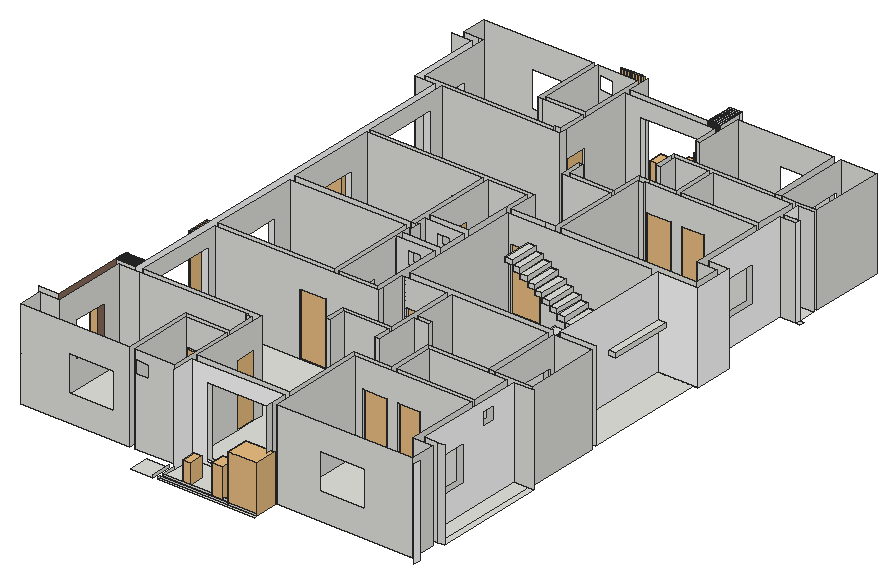
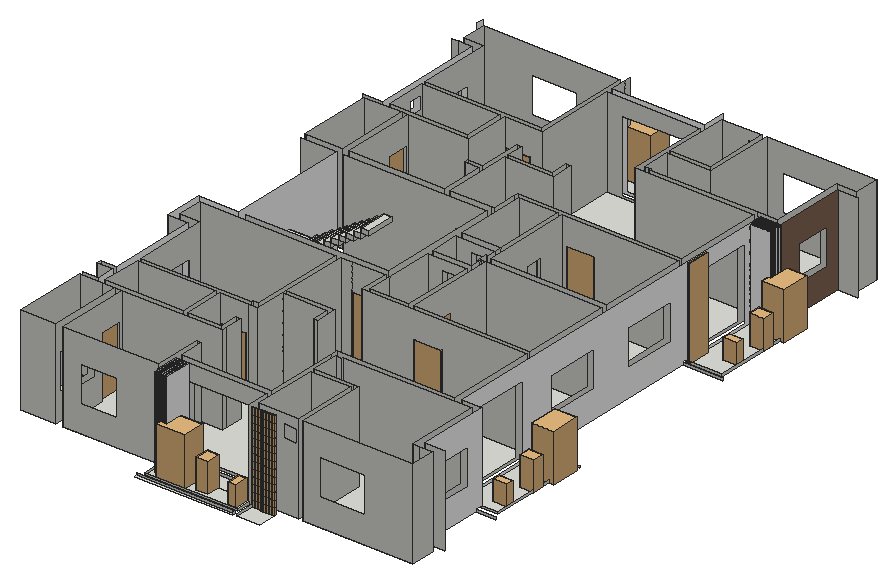
# SketchUp Ruby script. Lengths in inches.
U = 1.inch
M = Sketchup.active_model
def pt(a) = Geom::Point3d.new(a.map { |v| v * U })
def face(e, loops, mat)
  f = e.add_face(loops[0].map { |a| pt(a) })
  loops[1..].each { |l| e.add_face(l.map { |a| pt(a) }).erase! }
  f.material = f.back_material = mat if mat
  f
end
# faces: each face lists its corners as indices into pts; further lists are holes
def faces(e, pts, list, mat = nil) = list.each { |f| face(e, (f[0].is_a?(Array) ? f : [f]).map { |l| l.map { |i| pts[i] } }, mat) }
# xy, xz, yz: faces in a plane at the given z, y or x. An outline is a flat list of corners, or four numbers for a rectangle; further outlines are holes
def ring(l) = l.size == 4 ? [[l[0], l[1]], [l[2], l[1]], [l[2], l[3]], [l[0], l[3]]] : l.each_slice(2).to_a
def flat(e, list, mat, &to3) = list.each { |f| face(e, (f[0].is_a?(Array) ? f : [f]).map { |l| ring(l).map { |u, v| to3.(u, v) } }, mat) }
def xy(e, z, list, mat = nil) = flat(e, list, mat) { |x, y| [x, y, z] }
def xz(e, y, list, mat = nil) = flat(e, list, mat) { |x, z| [x, y, z] }
def yz(e, x, list, mat = nil) = flat(e, list, mat) { |y, z| [x, y, z] }
def lines(e, pts, list) = list.each { |a, b| e.add_line(pt(pts[a]), pt(pts[b])) }
# prism: a flat outline (further loops are holes) pulled along v
def prism(e, loops, v, mat = nil)
  f = face(e, loops, mat); d = Geom::Vector3d.new(v.map { |x| x * U })
  f.pushpull(f.normal.samedirection?(d) ? d.length : -d.length)
end
def box(e, o, s, mat = nil) = prism(e, [[o, [o[0] + s[0], o[1], o[2]], [o[0] + s[0], o[1] + s[1], o[2]], [o[0], o[1] + s[1], o[2]]]], [0, 0, s[2]], mat)
def at(x, y, z, deg = 0) = Geom::Transformation.translation(pt([x, y, z])) * Geom::Transformation.rotation(ORIGIN, Z_AXIS, deg.degrees)
def axes(o, x, y, z) = Geom::Transformation.new([*x, 0, *y, 0, *z, 0, *pt(o).to_a, 1])
def part(name) = M.definitions.add(name)
# library, detail: a bought-in or finely detailed component or shape, given as its bounding box
def library(name, o, s) = part(name).tap { |d| box(d.entities, o, s) }
def detail(e, o, s) = box(e.add_group.entities, o, s)
def put(e, d, t, mat = nil) = e.add_instance(d, t).tap { |i| i.material = mat if mat }
def group(e, t, mat = nil) = e.add_group.tap { |g| g.transformation = t; g.material = mat if mat }.entities
root = M.entities
M.materials.add("Manhattan Creative Coating ML 1016B 24.75cm").color = [255, 255, 255]
M.materials.add("Wintan - wpa36452 29.79cm").color = [255, 255, 255]
M.materials.add("Wood Planks C01 100cm").color = [136, 107, 89]
c1 = library("Door 243 053",[-21.6,-2.79,-0.07],[43.2,5.58,82.64])
c2 = library("Potted Plant 13",[-10,-7.28,0],[18.93,15.17,39.22])
c3 = library("Potted Plant 50-12",[-6.11,-5.26,0],[11.24,10.56,13.41])
c4 = library("Potted Plant 02",[-16.98,-19.78,0],[30.04,38.68,37.52])
c5 = part("Rectangular column")
box(c5.entities,[0,16,0],[27,1,119.8])
box(c5.entities,[0,3.56,0],[27,1,120])
box(c5.entities,[0,1.78,0],[27,1,120])
box(c5.entities,[0,14.22,0],[27,1,119.8])
box(c5.entities,[0,5.33,0],[27,1,120])
box(c5.entities,[0,7.11,0],[27,1,120])
box(c5.entities,[0,10.67,0],[27,1,120.2])
box(c5.entities,[0,12.44,0],[27,1,119.8])
box(c5.entities,[0,0,0],[27,1,120])
xy(c5.entities,0,[[0,8.89,27,9.89]])
xy(c5.entities,120,[[0,8.89,27,9.89]])
xz(c5.entities,8.89,[[0,0,27,120]])
xz(c5.entities,9.89,[[0,0,27,120]])
yz(c5.entities,0,[[8.89,0,9.89,120]],"Wintan - wpa36452 29.79cm")
yz(c5.entities,27,[[8.89,0,9.89,120]])
c6 = part("Stair tread \#1")
box(c6.entities,[0,0,0],[10,39,7])
c7 = part("Stair tread")
box(c7.entities,[0,0,0],[10,39,7])
c8 = part("Group\#9")
box(c8.entities,[100,0,63],[49,84,7])
box(c8.entities,[0,45,0],[20,39,7])
put(c8.entities,c6,at(50,45,28))
put(c8.entities,c6,at(20,45,7))
put(c8.entities,c6,at(90,45,56))
put(c8.entities,c6,at(70,45,42))
put(c8.entities,c6,at(40,45,21))
put(c8.entities,c6,at(60,45,35))
put(c8.entities,c6,at(30,45,14))
put(c8.entities,c6,at(80,45,49))
put(c8.entities,c7,at(90,0,70))
put(c8.entities,c7,at(10,0,126))
put(c8.entities,c7,at(60,0,91))
put(c8.entities,c7,at(30,0,112))
put(c8.entities,c7,at(50,0,98))
put(c8.entities,c7,at(70,0,84))
put(c8.entities,c7,at(80,0,77))
put(c8.entities,c7,at(40,0,105))
put(c8.entities,c7,at(0,0,133))
put(c8.entities,c7,at(20,0,119))
c9 = part("Decorative grille insert")
p = [[0.961,0,5],[0.961,0,4.995]]
lines(c9.entities,p,[[0,1]])
detail(c9.entities,[0,0,0],[4.12,1.8,10])
c10 = part("Group\#25")
put(c10.entities,c9,at(0,0,0))
put(c10.entities,c9,at(4.12,0,0))
put(c10.entities,c9,at(8.24,0,0))
put(c10.entities,c9,at(12.36,0,0))
put(c10.entities,c9,at(16.48,0,0))
put(c10.entities,c9,at(20.61,0,0))
put(c10.entities,c9,at(24.73,0,0))
put(c10.entities,c9,at(28.85,0,0))
put(c10.entities,c9,at(0,0,10))
put(c10.entities,c9,at(28.85,0,10))
put(c10.entities,c9,at(24.73,0,10))
put(c10.entities,c9,at(20.61,0,10))
put(c10.entities,c9,at(12.36,0,10))
put(c10.entities,c9,at(16.48,0,10))
put(c10.entities,c9,at(4.12,0,10))
put(c10.entities,c9,at(8.24,0,10))
put(c10.entities,c9,at(0,0,20))
put(c10.entities,c9,at(28.85,0,20))
put(c10.entities,c9,at(24.73,0,20))
put(c10.entities,c9,at(20.61,0,20))
put(c10.entities,c9,at(12.36,0,20))
put(c10.entities,c9,at(16.48,0,20))
put(c10.entities,c9,at(4.12,0,20))
put(c10.entities,c9,at(8.24,0,20))
put(c10.entities,c9,at(0,0,30))
put(c10.entities,c9,at(28.85,0,30))
put(c10.entities,c9,at(24.73,0,30))
put(c10.entities,c9,at(20.61,0,30))
put(c10.entities,c9,at(12.36,0,30))
put(c10.entities,c9,at(16.48,0,30))
put(c10.entities,c9,at(4.12,0,30))
put(c10.entities,c9,at(8.24,0,30))
put(c10.entities,c9,at(0,0,40))
put(c10.entities,c9,at(28.85,0,40))
put(c10.entities,c9,at(24.73,0,40))
put(c10.entities,c9,at(20.61,0,40))
put(c10.entities,c9,at(12.36,0,40))
put(c10.entities,c9,at(16.48,0,40))
put(c10.entities,c9,at(4.12,0,40))
put(c10.entities,c9,at(8.24,0,40))
put(c10.entities,c9,at(0,0,50))
put(c10.entities,c9,at(28.85,0,50))
put(c10.entities,c9,at(24.73,0,50))
put(c10.entities,c9,at(20.61,0,50))
put(c10.entities,c9,at(12.36,0,50))
put(c10.entities,c9,at(16.48,0,50))
put(c10.entities,c9,at(4.12,0,50))
put(c10.entities,c9,at(8.24,0,50))
put(c10.entities,c9,at(0,0,60))
put(c10.entities,c9,at(28.85,0,60))
put(c10.entities,c9,at(24.73,0,60))
put(c10.entities,c9,at(20.61,0,60))
put(c10.entities,c9,at(12.36,0,60))
put(c10.entities,c9,at(16.48,0,60))
put(c10.entities,c9,at(4.12,0,60))
put(c10.entities,c9,at(8.24,0,60))
put(c10.entities,c9,at(0,0,70))
put(c10.entities,c9,at(28.85,0,70))
put(c10.entities,c9,at(24.73,0,70))
put(c10.entities,c9,at(20.61,0,70))
put(c10.entities,c9,at(12.36,0,70))
put(c10.entities,c9,at(16.48,0,70))
put(c10.entities,c9,at(4.12,0,70))
put(c10.entities,c9,at(8.24,0,70))
put(c10.entities,c9,at(0,0,80))
put(c10.entities,c9,at(28.85,0,80))
put(c10.entities,c9,at(24.73,0,80))
put(c10.entities,c9,at(20.61,0,80))
put(c10.entities,c9,at(12.36,0,80))
put(c10.entities,c9,at(16.48,0,80))
put(c10.entities,c9,at(4.12,0,80))
put(c10.entities,c9,at(8.24,0,80))
put(c10.entities,c9,at(0,0,90))
put(c10.entities,c9,at(28.85,0,90))
put(c10.entities,c9,at(24.73,0,90))
put(c10.entities,c9,at(20.61,0,90))
put(c10.entities,c9,at(12.36,0,90))
put(c10.entities,c9,at(16.48,0,90))
put(c10.entities,c9,at(4.12,0,90))
put(c10.entities,c9,at(8.24,0,90))
put(c10.entities,c9,at(0,0,100))
put(c10.entities,c9,at(28.85,0,100))
put(c10.entities,c9,at(24.73,0,100))
put(c10.entities,c9,at(20.61,0,100))
put(c10.entities,c9,at(12.36,0,100))
put(c10.entities,c9,at(16.48,0,100))
put(c10.entities,c9,at(4.12,0,100))
put(c10.entities,c9,at(8.24,0,100))
put(c10.entities,c9,at(0,0,110))
put(c10.entities,c9,at(28.85,0,110))
put(c10.entities,c9,at(24.73,0,110))
put(c10.entities,c9,at(20.61,0,110))
put(c10.entities,c9,at(12.36,0,110))
put(c10.entities,c9,at(16.48,0,110))
put(c10.entities,c9,at(4.12,0,110))
put(c10.entities,c9,at(8.24,0,110))
put(c10.entities,c9,at(0,0,120))
put(c10.entities,c9,at(28.85,0,120))
put(c10.entities,c9,at(24.73,0,120))
put(c10.entities,c9,at(20.61,0,120))
put(c10.entities,c9,at(12.36,0,120))
put(c10.entities,c9,at(16.48,0,120))
put(c10.entities,c9,at(4.12,0,120))
put(c10.entities,c9,at(8.24,0,120))
c11 = library("Group1606\#2",[0.89,0.19,0],[2.1,4.18,2.5])
xy(root,126,[[1975.05,473.67,2005.02,500.67],[2011.02,473.67,2141.52,476.67],[2011.02,482.67,2135.52,530.62],[1798.02,509.67,1945.02,509.67,1945.02,602.67,1954.02,602.67,1954.02,596.67,1951.02,596.67,1951.02,509.67,2005.02,509.67,2005.02,596.67,1978.02,596.67,1978.02,602.67,2005.02,602.67,2005.02,605.67,2011.02,605.67,2011.02,635.67,2005.02,635.67,2005.02,638.67,1997.02,638.67,1997.02,641.67,1825.02,641.67,1825.02,542.67,1798.02,542.67],[2141.52,509.67,2324.52,509.67,2324.52,542.67,2297.52,542.67,2297.52,641.67,2228.52,641.67,2228.52,647.67,2198.52,647.67,2198.52,641.67,2184.02,641.67,2184.02,647.67,2152.02,647.67,2152.02,641.67,2141.52,641.67],
  [2011.02,539.67,2135.52,539.67,2135.52,647.67,2186.52,647.67,2186.52,707.67,2267.52,707.67,2267.52,710.67,2276.52,710.67,2276.52,740.67,2267.52,740.67,2267.52,806.67,2138.52,806.67,2138.52,749.67,2158.52,749.67,2158.52,743.67,2138.52,743.67,2138.52,686.67,2132.52,686.67,2132.52,709.17,2072.52,709.17,2072.52,686.67,2066.52,686.67,2066.52,715.17,2132.52,715.17,2132.52,806.67,2117.52,806.67,2117.52,815.67,2078.52,815.67,2078.52,806.67,2072.52,806.67,2072.52,767.67,1852.02,767.67,1852.02,647.67,2011.02,647.67],[2306.52,551.67,2324.52,701.67],[2324.52,551.67,2333.52,701.67],[1795.02,643.17,1816.02,643.17,1816.02,647.67,1843.02,647.67,1843.02,772.17,1795.02,772.17],[2192.52,647.67,2297.52,701.67],
  [2066.52,686.67,2072.52,686.67,2072.52,709.17,2132.52,709.17,2132.52,686.67,2138.52,686.67,2138.52,743.67,2158.52,743.67,2158.52,749.67,2138.52,749.67,2138.52,806.67,2132.52,806.67,2132.52,715.17,2066.52,715.17],[2276.52,707.67,2324.52,806.67],[2324.52,707.67,2327.52,806.67],[1966.02,767.67,2002.02,767.67,2002.02,773.67,2008.02,773.67,2008.02,809.67,2014.02,809.67,2014.02,833.67,2008.02,833.67,2008.02,893.67,1852.02,893.67,1852.02,773.67,1966.02,773.67],[2014.02,773.67,2066.52,869.67],
  [2066.52,806.67,2075.52,806.67,2075.52,980.67,2078.52,980.67,2078.52,989.67,2072.52,989.67,2072.52,1028.67,2002.02,1028.67,2002.02,1022.67,2008.02,1022.67,2008.02,986.67,2014.02,986.67,2014.02,1022.67,2066.52,1022.67,2066.52,926.67,2014.02,926.67,2014.02,962.67,2008.02,962.67,2008.02,902.67,2014.02,902.67,2014.02,917.67,2066.52,917.67,2066.52,878.67,2014.02,878.67,2014.02,869.67,2066.52,869.67],[2075.52,815.67,2207.52,815.67,2207.52,887.67,2267.52,887.67,2267.52,896.67,2138.52,896.67,2138.52,980.67,2117.52,980.67,2117.52,989.67,2078.52,989.67,2078.52,980.67,2075.52,980.67],[2276.52,815.67,2324.52,980.67],[2014.02,878.67,2066.52,878.67,2066.52,917.67,2014.02,917.67,2014.02,905.17,2017.02,905.17,2017.02,891.17,2014.02,891.17],[2143.41,896.68,2143.67,896.68,2143.92,896.76,2144.15,896.89,2144.33,897.08,2144.45,897.31,2144.52,897.56,2144.51,897.82,2144.44,898.07,2144.31,898.3,2144.12,898.48,2143.89,898.6,2143.64,898.67,2143.38,898.66,2143.125,898.59,2142.9,898.46,2142.72,898.27,2142.59,898.04,2142.53,897.79,2142.53,897.53,2142.61,897.28,2142.74,897.05,2142.93,896.87,2143.16,896.74],
  [1852.02,902.67,2008.02,902.67,2008.02,962.67,2014.02,962.67,2014.02,986.67,2008.02,986.67,2008.02,1022.67,2002.02,1022.67,2002.02,1028.67,1966.02,1028.67,1966.02,1022.67,1852.02,1022.67],[2014.02,926.67,2066.52,1022.67],[2143.41,933.68,2143.67,933.68,2143.92,933.76,2144.15,933.89,2144.33,934.08,2144.45,934.31,2144.52,934.56,2144.51,934.82,2144.44,935.07,2144.31,935.3,2144.12,935.48,2143.89,935.6,2143.64,935.67,2143.38,935.66,2143.125,935.59,2142.9,935.46,2142.72,935.27,2142.59,935.04,2142.53,934.79,2142.53,934.53,2142.61,934.28,2142.74,934.05,2142.93,933.87,2143.16,933.74],[2132.52,980.67,2330.52,980.67,2330.52,1022.67,2321.52,1022.67,2321.52,989.67,2138.52,989.67,2138.52,1118.67,2132.52,1118.67],[2072.52,989.67,2132.52,989.67,2132.52,1081.17,2066.52,1081.17,2066.52,1109.67,2072.52,1109.67,2072.52,1087.17,2132.52,1087.17,2132.52,1127.67,2149.02,1127.67,2149.02,1121.67,2146.52,1121.67,2146.52,1118.67,2138.52,1118.67,2138.52,989.67,2321.52,989.67,2321.52,1022.67,2294.52,1022.67,2294.52,1121.67,2225.52,1121.67,2225.52,1127.67,2195.52,1127.67,2195.52,1121.67,2181.02,1121.67,2181.02,1127.67,2183.52,1127.67,2183.52,1181.67,2138.52,1181.67,2138.52,1157.67,2132.52,1157.67,2132.52,1187.67,2267.52,1187.67,2267.52,1190.67,2276.52,1190.67,2276.52,1220.67,2267.52,1220.67,2267.52,1286.67,2138.52,1286.67,2138.52,1223.67,2132.52,1223.67,2132.52,1256.67,2011.02,1256.67,2011.02,1148.67,1852.02,1148.67,1852.02,1028.67,2072.52,1028.67],
  [1852.02,1022.67,1966.02,1028.67],[2294.52,1022.67,2330.52,1022.67,2330.52,1031.67,2303.52,1031.67,2303.52,1151.7,2324.52,1151.7,2324.52,1157.7,2303.52,1157.7,2303.52,1181.67,2294.52,1181.67],[1795.02,1024.17,1843.02,1148.67],[2189.52,1127.67,2294.52,1181.67],[2324.52,1151.7,2330.52,1157.7],
  [1825.02,1154.67,1997.02,1154.67,1997.02,1157.67,2005.02,1157.67,2005.02,1160.17,2011.02,1160.17,2011.02,1190.17,2005.02,1190.17,2005.02,1193.67,1978.02,1193.67,1978.02,1199.67,1954.02,1199.67,1954.02,1193.67,1945.02,1193.67,1945.02,1286.67,1798.02,1286.67,1798.02,1253.67,1825.02,1253.67],[2303.52,1157.7,2324.52,1181.67],[2276.52,1187.67,2324.52,1286.67],[1951.02,1199.67,2005.02,1286.67],[2011.02,1265.67,2132.52,1286.67],
  [2011.02,1286.67,2132.52,1286.67,2132.52,1295.67,2135.52,1295.67,2135.52,1313.67,2011.02,1313.67],[1975.05,1295.67,2005.02,1322.67],[2011.02,1319.67,2141.52,1322.67]])
xz(root,476.67,[[2011.02,126,2141.52,129]])
xz(root,482.67,[[2011.02,126,2135.52,129]])
xz(root,509.67,[[[1798.02,126,1945.02,246],[1863.02,162,1923.02,210]],[[1951.02,126,2005.02,246],[1953.02,216,1970.52,234]],[[2141.52,126,2324.52,246],[2199.52,162,2259.52,210]]])
xz(root,530.62,[[[2011.02,126,2135.52,246],[2031.27,129,2115.27,225]]],"Manhattan Creative Coating ML 1016B 24.75cm")
xz(root,539.67,[[[2011.02,126,2135.52,246],[2031.27,129,2115.27,225]]])
xz(root,542.67,[[1798.02,126,1825.02,246],[2297.52,126,2324.52,246]])
xz(root,551.67,[[1789.02,126,1816.02,246],[2306.52,126,2324.52,246],[2324.52,126,2333.52,246]])
xz(root,596.67,[[1951.02,126,1954.02,126,1954.02,210,1978.02,210,1978.02,126,2005.02,126,2005.02,246,1951.02,246]])
xz(root,602.67,[[1945.02,126,1945.02,246,2005.02,246,2005.02,126,1978.02,126,1978.02,210,1954.02,210,1954.02,126]])
xz(root,605.67,[[2005.02,126,2011.02,210]])
xz(root,635.67,[[2005.02,126,2011.02,210]])
xz(root,637.17,[[1789.02,126,1816.02,129]])
xz(root,638.67,[[1997.02,126,2005.02,246]])
xz(root,641.67,[[1825.02,126,1852.02,246],[1852.02,126,1997.02,246],[2141.52,126,2152.02,126,2152.02,210,2184.02,210,2184.02,126,2198.52,126,2198.52,210,2228.52,210,2228.52,126,2297.52,126,2297.52,246,2141.52,246]])
xz(root,643.17,[[1795.02,126,1816.02,129]])
xz(root,647.67,[[1816.02,126,1843.02,246],[1852.02,126,2011.02,246],[2135.52,126,2135.52,246,2186.52,246,2186.52,126,2184.02,126,2184.02,210,2152.02,210,2152.02,126],[2192.52,126,2192.52,246,2297.52,246,2297.52,126,2228.52,126,2228.52,210,2198.52,210,2198.52,126]])
xz(root,686.67,[[2066.52,126,2072.52,246],[2132.52,126,2138.52,246]])
xz(root,701.67,[[2192.52,126,2297.52,246],[2306.52,126,2333.52,246]])
xz(root,707.67,[[2186.52,126,2267.52,246],[2267.52,126,2276.52,246],[2276.52,126,2327.52,246]])
xz(root,709.17,[[2072.52,126,2132.52,246]])
xz(root,710.67,[[2267.52,126,2276.52,210]])
xz(root,715.17,[[2066.52,126,2132.52,246]])
xz(root,740.67,[[2267.52,126,2276.52,210]])
xz(root,743.67,[[2138.52,126,2158.52,246]])
xz(root,749.67,[[2138.52,126,2158.52,246]])
xz(root,767.67,[[1852.02,126,1966.02,126,1966.02,210,2002.02,210,2002.02,126,2072.52,126,2072.52,246,1852.02,246]])
xz(root,772.17,[[1795.02,126,1843.02,129]])
xz(root,773.67,[[1852.02,126,1852.02,246,2008.02,246,2008.02,126,2002.02,126,2002.02,210,1966.02,210,1966.02,126],[2014.02,126,2066.52,246]])
xz(root,778.17,[[1789.02,126,1843.02,129]])
xz(root,806.67,[[2072.52,126,2075.52,246],[2075.52,126,2078.52,126,2078.52,210,2117.52,210,2117.52,126,2132.52,126,2132.52,246,2075.52,246],[2138.52,126,2267.52,246],[2276.52,126,2324.52,246],[2324.52,126,2327.52,246]])
xz(root,809.67,[[2008.02,126,2014.02,210]])
xz(root,815.67,[[2075.52,126,2075.52,246,2267.52,246,2267.52,126,2117.52,126,2117.52,210,2078.52,210,2078.52,126],[2276.52,126,2324.52,246]])
xz(root,833.67,[[2008.02,126,2014.02,210]])
xz(root,869.67,[[[2014.02,126,2066.52,246],[2029.77,216,2047.27,234]]])
xz(root,878.67,[[[2014.02,126,2066.52,246],[2029.77,216,2047.27,234]]])
xz(root,891.17,[[2014.02,126,2017.02,246]])
xz(root,893.67,[[1852.02,126,2008.02,246]])
xz(root,902.67,[[1852.02,126,2008.02,246],[2008.02,126,2014.02,246]])
xz(root,905.17,[[2014.02,126,2017.02,246]])
xz(root,917.67,[[[2014.02,126,2066.52,246],[2029.77,216,2047.27,234]]])
xz(root,926.67,[[[2014.02,126,2066.52,246],[2029.77,216,2047.27,234]]])
xz(root,962.67,[[2008.02,126,2014.02,210]])
xz(root,980.67,[[2075.52,126,2078.52,126,2078.52,210,2117.52,210,2117.52,126,2267.52,126,2267.52,246,2075.52,246]])
xz(root,980.67,[[2276.52,126,2330.52,246]],"Manhattan Creative Coating ML 1016B 24.75cm")
xz(root,986.67,[[2008.02,126,2014.02,210]])
xz(root,989.67,[[2072.52,126,2072.52,246,2117.52,246,2117.52,210,2078.52,210,2078.52,126],[2117.52,126,2132.52,246],[2138.52,126,2321.52,246]])
xz(root,1018.17,[[1789.02,126,1843.02,129]])
xz(root,1022.67,[[1852.02,126,1966.02,126,1966.02,210,2002.02,210,2002.02,126,2008.02,126,2008.02,246,1852.02,246],[2014.02,126,2066.52,246],[2294.52,126,2321.52,246]])
xz(root,1024.17,[[1795.02,126,1843.02,129]])
xz(root,1028.67,[[1852.02,126,1852.02,246,2072.52,246,2072.52,126,2002.02,126,2002.02,210,1966.02,210,1966.02,126]])
xz(root,1031.67,[[2303.52,126,2330.52,246]])
xz(root,1081.17,[[2066.52,126,2132.52,246]])
xz(root,1087.17,[[2072.52,126,2132.52,246]])
xz(root,1109.67,[[2066.52,126,2072.52,246]])
xz(root,1118.67,[[2138.52,126,2146.52,246]])
xz(root,1121.67,[[2146.52,126,2149.02,126,2149.02,210,2181.02,210,2181.02,126,2195.52,126,2195.52,210,2225.52,210,2225.52,126,2294.52,126,2294.52,246,2146.52,246]])
xz(root,1127.67,[[2132.52,126,2146.52,246],[2146.52,126,2146.52,246,2183.52,246,2183.52,126,2181.02,126,2181.02,210,2149.02,210,2149.02,126],[2189.52,126,2189.52,246,2294.52,246,2294.52,126,2225.52,126,2225.52,210,2195.52,210,2195.52,126]])
xz(root,1148.67,[[1795.02,126,1816.02,129],[1816.02,126,1843.02,246],[1852.02,126,2011.02,246]])
xz(root,1151.7,[[2303.52,126,2324.52,246]])
xz(root,1154.67,[[1825.02,126,1997.02,246]])
xz(root,1157.67,[[1997.02,126,2005.02,246],[2132.52,126,2138.52,246]])
xz(root,1157.7,[[2303.52,126,2324.52,246]])
xz(root,1159.17,[[1789.02,126,1816.02,129]])
xz(root,1160.17,[[2005.02,126,2011.02,210]])
xz(root,1181.67,[[2138.52,126,2183.52,246],[2189.52,126,2294.52,246],[2303.52,126,2324.52,246]])
xz(root,1187.67,[[2132.52,126,2267.52,246],[2267.52,126,2276.52,246],[2276.52,126,2294.52,246],[2294.52,126,2324.52,246]])
xz(root,1190.17,[[2005.02,126,2011.02,210]])
xz(root,1190.67,[[2267.52,126,2276.52,210]])
xz(root,1193.67,[[1945.02,126,1951.02,246],[1951.02,126,1954.02,126,1954.02,210,1978.02,210,1978.02,126,2005.02,126,2005.02,246,1951.02,246]])
xz(root,1199.67,[[1951.02,126,1951.02,246,2005.02,246,2005.02,126,1978.02,126,1978.02,210,1954.02,210,1954.02,126]])
xz(root,1220.67,[[2267.52,126,2276.52,210]])
xz(root,1223.67,[[2132.52,126,2138.52,246]])
xz(root,1244.67,[[1789.02,126,1816.02,246]])
xz(root,1253.67,[[1798.02,126,1816.02,246],[1816.02,126,1825.02,246]])
xz(root,1256.67,[[[2011.02,126,2132.52,246],[2031.27,129,2115.27,225]]])
xz(root,1265.67,[[[2011.02,126,2132.52,246],[2031.27,129,2115.27,225]]])
xz(root,1286.67,[[[1798.02,126,1945.02,246],[1863.02,162,1923.02,210]],[[1951.02,126,2005.02,246],[1953.02,216,1970.52,234]],[[2138.52,126,2267.52,246],[2195.52,162,2243.52,210]],[2276.52,126,2324.52,246]])
xz(root,1313.67,[[2011.02,126,2135.52,129]])
xz(root,1319.67,[[2011.02,126,2141.52,129]])
yz(root,1795.02,[[643.17,126,772.17,129],[1024.17,126,1148.67,129]])
yz(root,1798.02,[[509.67,126,542.67,246],[1253.67,126,1286.67,246]])
yz(root,1816.02,[[[1159.17,126,1159.17,129,1148.67,129,1148.67,246,1244.67,246,1244.67,126],[1172.67,162,1220.67,210]]],"Manhattan Creative Coating ML 1016B 24.75cm")
yz(root,1816.02,[[[551.67,126,551.67,246,647.67,246,647.67,126,643.17,126,643.17,129,637.17,129,637.17,126],[569.57,162,617.57,210]]],"Wood Planks C01 100cm")
yz(root,1825.02,[[[542.67,126,641.67,246],[569.57,162,617.57,210]],[[1154.67,126,1253.67,246],[1172.67,162,1220.67,210]]])
yz(root,1843.02,[[[647.67,126,647.67,246,1148.67,246,1148.67,126,1024.17,126,1024.17,129,1018.17,129,1018.17,126,778.17,126,778.17,129,772.17,129,772.17,126],[1046.67,129,1130.67,225],[673.67,129,757.67,225],[926.67,162,998.67,210],[797.67,162,869.67,210]]],"Manhattan Creative Coating ML 1016B 24.75cm")
yz(root,1852.02,[[[647.67,126,767.67,246],[673.67,129,757.67,225]],[[773.67,126,893.67,246],[797.67,162,869.67,210]],[[902.67,126,1022.67,246],[926.67,162,998.67,210]],[[1028.67,126,1148.67,246],[1046.67,129,1130.67,225]]])
yz(root,1945.02,[[509.67,126,602.67,246],[1193.67,126,1286.67,246]])
yz(root,1951.02,[[509.67,126,596.67,246],[1199.67,126,1286.67,246]])
yz(root,1954.02,[[596.67,126,602.67,210],[1193.67,126,1199.67,210]])
yz(root,1966.02,[[767.67,126,773.67,210],[1022.67,126,1028.67,210]])
yz(root,1978.02,[[596.67,126,602.67,210],[1193.67,126,1199.67,210]])
yz(root,1997.02,[[638.67,126,641.67,246],[1154.67,126,1157.67,246]])
yz(root,2002.02,[[767.67,126,773.67,210],[1022.67,126,1028.67,210]])
yz(root,2005.02,[[473.67,126,500.67,129],[509.67,126,596.67,246],[602.67,126,602.67,246,638.67,246,638.67,126,635.67,126,635.67,210,605.67,210,605.67,126],[1157.67,126,1157.67,246,1193.67,246,1193.67,126,1190.17,126,1190.17,210,1160.17,210,1160.17,126],[1199.67,126,1286.67,246],
  [1295.67,126,1322.67,129]])
yz(root,2008.02,[[773.67,126,773.67,246,893.67,246,893.67,126,833.67,126,833.67,210,809.67,210,809.67,126],[902.67,126,902.67,246,1022.67,246,1022.67,126,986.67,126,986.67,210,962.67,210,962.67,126]])
yz(root,2011.02,[[473.67,126,476.67,129],[482.67,126,500.67,129],[539.67,126,605.67,126,605.67,210,635.67,210,635.67,126,647.67,126,647.67,246,539.67,246],[1148.67,126,1157.67,246],[1157.67,126,1160.17,126,1160.17,210,1190.17,210,1190.17,126,1256.67,126,1256.67,246,1157.67,246],
  [1265.67,126,1295.67,246],[1295.67,126,1313.67,129],[1319.67,126,1322.67,129]])
yz(root,2011.02,[[500.67,126,530.62,246]],"Manhattan Creative Coating ML 1016B 24.75cm")
yz(root,2014.02,[[773.67,126,809.67,126,809.67,210,833.67,210,833.67,126,869.67,126,869.67,246,773.67,246],[869.67,126,878.67,246],[878.67,126,891.17,246],[902.67,126,905.17,246],[905.17,126,917.67,246],
  [926.67,126,962.67,126,962.67,210,986.67,210,986.67,126,1022.67,126,1022.67,246,926.67,246]])
yz(root,2017.02,[[891.17,126,905.17,246]])
yz(root,2066.52,[[686.67,126,715.17,246],[773.67,126,869.67,246],[878.67,126,917.67,246],[926.67,126,989.67,246],[989.67,126,1022.67,246],
  [1081.17,126,1109.67,246]])
yz(root,2072.52,[[686.67,126,709.17,246],[767.67,126,773.67,246],[773.67,126,806.67,246],[989.67,126,1028.67,246],[1087.17,126,1109.67,246]])
yz(root,2075.52,[[815.67,126,980.67,246]])
yz(root,2078.52,[[806.67,126,815.67,210],[980.67,126,989.67,210]])
yz(root,2117.52,[[806.67,126,815.67,210],[980.67,126,989.67,210]])
yz(root,2132.52,[[686.67,126,709.17,246],[715.17,126,806.67,246],[989.67,126,1081.17,246],[1081.17,126,1087.17,246],[1087.17,126,1127.67,246],
  [1157.67,126,1181.67,246],[1181.67,126,1187.67,246],[1223.67,126,1256.67,246],[1265.67,126,1295.67,246]])
yz(root,2135.52,[[482.67,126,500.67,129],[500.67,126,509.67,246],[509.67,126,530.62,246],[539.67,126,647.67,246],[1295.67,126,1313.67,129]])
yz(root,2138.52,[[686.67,126,743.67,246],[749.67,126,806.67,246],[989.67,126,1118.67,246],[1157.67,126,1181.67,246],[1223.67,126,1286.67,246]])
yz(root,2141.52,[[509.67,126,641.67,246]])
yz(root,2146.52,[[1118.67,126,1121.67,246]])
yz(root,2149.02,[[1121.67,126,1127.67,210]])
yz(root,2152.02,[[641.67,126,647.67,210]])
yz(root,2158.52,[[743.67,126,749.67,246]])
yz(root,2181.02,[[1121.67,126,1127.67,210]])
yz(root,2183.52,[[1127.67,126,1181.67,246]])
yz(root,2184.02,[[641.67,126,647.67,210]])
yz(root,2186.52,[[647.67,126,707.67,246]])
yz(root,2189.52,[[1127.67,126,1181.67,246]])
yz(root,2192.52,[[647.67,126,701.67,246]])
yz(root,2195.52,[[1121.67,126,1127.67,210]])
yz(root,2198.52,[[641.67,126,647.67,210]])
yz(root,2225.52,[[1121.67,126,1127.67,210]])
yz(root,2228.52,[[641.67,126,647.67,210]])
yz(root,2267.52,[[[707.67,126,707.67,246,806.67,246,806.67,126,740.67,126,740.67,210,710.67,210,710.67,126],[752.67,162,800.67,210]],[[1187.67,126,1187.67,246,1286.67,246,1286.67,126,1220.67,126,1220.67,210,1190.67,210,1190.67,126],[1232.67,162,1280.67,210]]])
yz(root,2276.52,[[[707.67,126,710.67,126,710.67,210,740.67,210,740.67,126,806.67,126,806.67,246,707.67,246],[752.67,162,800.67,210]],[[1187.67,126,1190.67,126,1190.67,210,1220.67,210,1220.67,126,1286.67,126,1286.67,246,1187.67,246],[1232.67,162,1280.67,210]]])
yz(root,2276.52,[[815.67,126,980.67,246]],"Manhattan Creative Coating ML 1016B 24.75cm")
yz(root,2294.52,[[[1022.67,126,1121.67,246],[1040.67,162,1106.67,210]],[[1127.67,126,1181.67,246],[1162.17,216,1179.67,234]]])
yz(root,2297.52,[[[542.67,126,641.67,246],[569.57,162,617.57,210]],[[647.67,126,701.67,246],[649.73,216,667.23,234]]])
yz(root,2303.52,[[[1031.67,126,1151.7,246],[1040.67,162,1106.67,210]],[[1157.7,126,1181.67,246],[1162.17,216,1179.67,234]]],"Manhattan Creative Coating ML 1016B 24.75cm")
yz(root,2306.52,[[[551.67,126,701.67,246],[569.57,162,617.57,210],[649.73,216,667.23,234]]],"Manhattan Creative Coating ML 1016B 24.75cm")
yz(root,2321.52,[[989.67,126,1022.67,246]])
yz(root,2324.52,[[509.67,126,542.67,246],[1187.67,126,1286.67,246]])
yz(root,2324.52,[[1151.7,126,1157.7,246]],"Manhattan Creative Coating ML 1016B 24.75cm")
yz(root,2327.52,[[707.67,126,806.67,246]])
yz(root,2330.52,[[980.67,126,1031.67,246]],"Manhattan Creative Coating ML 1016B 24.75cm")
yz(root,2333.52,[[500.67,126,509.67,246]],"Manhattan Creative Coating ML 1016B 24.75cm")
p = [[2138.52,896.67,126],[2138.52,980.67,126],[2267.52,980.67,126],[2267.52,896.67,126],[2138.52,896.67,126],[2138.52,980.67,126],
  [2267.52,980.67,126],[2267.52,896.67,126],[2297.52,641.67,126],[2297.52,647.67,126],[2143.35,500.67,126],[2141.52,500.67,126]]
lines(root,p,[[0,1],[1,2],[2,3],[3,0],[4,5],[5,6],[6,7],[7,4],[8,9],[10,11]])
put(root,c1,axes([2213.52,646.74,125.43],[0.69441,0,0],[0,0.74,0],[0,0,1.01843]))
put(root,c1,axes([2168.02,646.74,125.43],[0.7407,0,0],[0,0.74,0],[0,0,1.01843]))
put(root,c1,axes([2273.94,1205.63,125.86],[0,-0.69441,0],[0.74,0,0],[0,0,1.01843]))
put(root,c1,axes([1966.02,1196.98,125.91],[0.55552,0,0],[0,0.74,0],[0,0,1.01843]))
put(root,c1,axes([1984.02,771.84,125.91],[0.83329,0,0],[0,0.74,0],[0,0,1.01843]))
put(root,c1,axes([1984.02,1027.84,125.91],[0.83329,0,0],[0,0.74,0],[0,0,1.01843]))
put(root,c1,axes([1965.99,597.61,126],[-0.55696,0,0],[0,-1.07698,0],[0,0,1.01843]))
put(root,c2,at(2084.22,492.59,126,90))
put(root,c2,at(1803.85,1081.33,126))
put(root,c2,at(2066.61,1296.4375,126,90))
put(root,c3,axes([2040.7,496.15,126],[0,1.65,0],[-1,0,0],[0,0,2]))
put(root,c3,axes([1807.42,1124.84,126],[1.65,0,0],[0,1,0],[0,0,2]))
put(root,c2,at(1804.9375,694.48,126))
put(root,c4,axes([2121.74,493.66,126],[0,1,0],[-1,0,0],[0,0,1.71]))
put(root,c5,at(1816.02,647.67,126),"Wintan - wpa36452 29.79cm")
put(root,c3,axes([2023.09,1300,126],[0,1.65,0],[-1,0,0],[0,0,2]))
put(root,c1,axes([2097.77,811.09,126.07],[0.9143,0,0],[0,0.74,0],[0,0,1.01843]))
put(root,c1,axes([2097.77,985.74,126.07],[0.9143,0,0],[0,0.74,0],[0,0,1.01843]))
put(root,c8,axes([2138.52,896.67,126],[1,0,0],[0,1,0],[0,0,0.9]))
put(root,c1,axes([2210.52,1123.74,126.07],[0.69441,0,0],[0,0.74,0],[0,0,1.01843]))
put(root,c1,axes([2165.02,1123.74,126.07],[0.7407,0,0],[0,0.74,0],[0,0,1.01843]))
put(root,c1,axes([2004.96,1175.17,126.07],[0,-0.69441,0],[0.74,0,0],[0,0,1.01843]))
put(root,c1,axes([2011.02,974.68,126.07],[0,-0.55585,0],[1.07698,0,0],[0,0,1.01843]))
put(root,c1,axes([2006.02,620.3,126.07],[0,-0.71149,0],[1.07698,0,0],[0,0,1.01843]))
put(root,c10,axes([1975.05,1295.67,126],[0.90915,0,0],[0,1,0],[0,0,0.92482]))
put(root,c11,axes([1841.02,784.99,120.55],[0,-14.41,0],[0,0,28.70953],[-1,0,0]))
put(root,c5,axes([2132.52,1265.67,126],[0,1.33704,0],[-1,0,0],[0,0,0.99834]),"Wintan - wpa36452 29.79cm")
put(root,c1,axes([2274.59,725.67,126.07],[0,-0.69441,0],[0.74,0,0],[0,0,1.01843]))
put(root,c4,axes([1804.92,1043.8,126],[1,0,0],[0,1,0],[0,0,1.71]))
put(root,c4,axes([2104.14,1297.51,126],[0,1,0],[-1,0,0],[0,0,1.71]))
put(root,c3,axes([1808.5,738,126],[1.65,0,0],[0,1,0],[0,0,2]))
put(root,c4,axes([1806.01,656.95,126],[1,0,0],[0,1,0],[0,0,1.71]))
